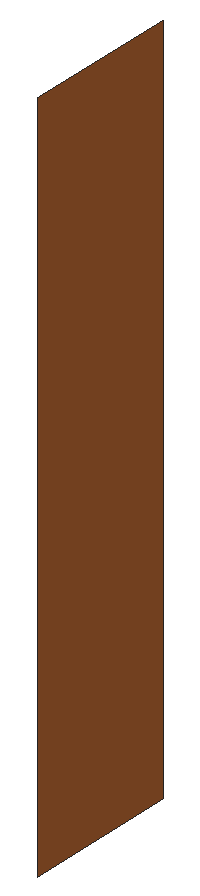
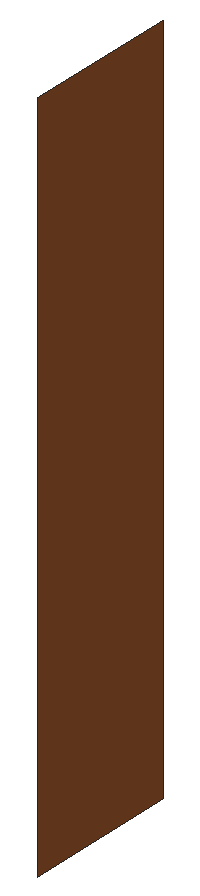
# SketchUp Ruby script. Lengths in inches.
U = 1.inch
M = Sketchup.active_model
def pt(a) = Geom::Point3d.new(a.map { |v| v * U })
def face(e, loops, mat)
  f = e.add_face(loops[0].map { |a| pt(a) })
  loops[1..].each { |l| e.add_face(l.map { |a| pt(a) }).erase! }
  f.material = f.back_material = mat if mat
  f
end
# faces: each face lists its corners as indices into pts; further lists are holes
def faces(e, pts, list, mat = nil) = list.each { |f| face(e, (f[0].is_a?(Array) ? f : [f]).map { |l| l.map { |i| pts[i] } }, mat) }
# xy, xz, yz: faces in a plane at the given z, y or x. An outline is a flat list of corners, or four numbers for a rectangle; further outlines are holes
def ring(l) = l.size == 4 ? [[l[0], l[1]], [l[2], l[1]], [l[2], l[3]], [l[0], l[3]]] : l.each_slice(2).to_a
def flat(e, list, mat, &to3) = list.each { |f| face(e, (f[0].is_a?(Array) ? f : [f]).map { |l| ring(l).map { |u, v| to3.(u, v) } }, mat) }
def xy(e, z, list, mat = nil) = flat(e, list, mat) { |x, y| [x, y, z] }
def xz(e, y, list, mat = nil) = flat(e, list, mat) { |x, z| [x, y, z] }
def yz(e, x, list, mat = nil) = flat(e, list, mat) { |y, z| [x, y, z] }
def lines(e, pts, list) = list.each { |a, b| e.add_line(pt(pts[a]), pt(pts[b])) }
# prism: a flat outline (further loops are holes) pulled along v
def prism(e, loops, v, mat = nil)
  f = face(e, loops, mat); d = Geom::Vector3d.new(v.map { |x| x * U })
  f.pushpull(f.normal.samedirection?(d) ? d.length : -d.length)
end
def box(e, o, s, mat = nil) = prism(e, [[o, [o[0] + s[0], o[1], o[2]], [o[0] + s[0], o[1] + s[1], o[2]], [o[0], o[1] + s[1], o[2]]]], [0, 0, s[2]], mat)
def at(x, y, z, deg = 0) = Geom::Transformation.translation(pt([x, y, z])) * Geom::Transformation.rotation(ORIGIN, Z_AXIS, deg.degrees)
def axes(o, x, y, z) = Geom::Transformation.new([*x, 0, *y, 0, *z, 0, *pt(o).to_a, 1])
def part(name) = M.definitions.add(name)
# library, detail: a bought-in or finely detailed component or shape, given as its bounding box
def library(name, o, s) = part(name).tap { |d| box(d.entities, o, s) }
def detail(e, o, s) = box(e.add_group.entities, o, s)
def put(e, d, t, mat = nil) = e.add_instance(d, t).tap { |i| i.material = mat if mat }
def group(e, t, mat = nil) = e.add_group.tap { |g| g.transformation = t; g.material = mat if mat }.entities
root = M.entities
M.materials.add("[Wood Cherry Original]1").color = [152, 86, 42]
yz(root,441.13,[[178.92,43.94,184.11,66.97]],"[Wood Cherry Original]1")
